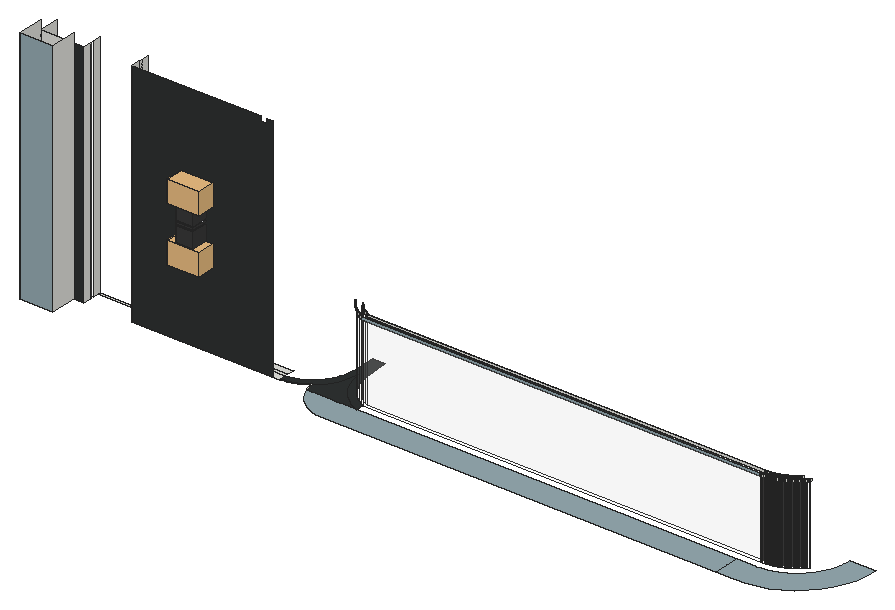
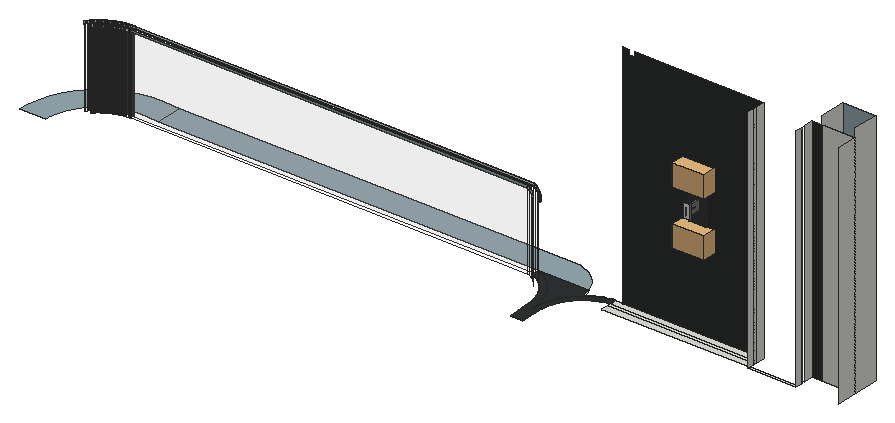
# SketchUp Ruby script. Lengths in inches.
U = 1.inch
M = Sketchup.active_model
def pt(a) = Geom::Point3d.new(a.map { |v| v * U })
def face(e, loops, mat)
  f = e.add_face(loops[0].map { |a| pt(a) })
  loops[1..].each { |l| e.add_face(l.map { |a| pt(a) }).erase! }
  f.material = f.back_material = mat if mat
  f
end
# faces: each face lists its corners as indices into pts; further lists are holes
def faces(e, pts, list, mat = nil) = list.each { |f| face(e, (f[0].is_a?(Array) ? f : [f]).map { |l| l.map { |i| pts[i] } }, mat) }
# xy, xz, yz: faces in a plane at the given z, y or x. An outline is a flat list of corners, or four numbers for a rectangle; further outlines are holes
def ring(l) = l.size == 4 ? [[l[0], l[1]], [l[2], l[1]], [l[2], l[3]], [l[0], l[3]]] : l.each_slice(2).to_a
def flat(e, list, mat, &to3) = list.each { |f| face(e, (f[0].is_a?(Array) ? f : [f]).map { |l| ring(l).map { |u, v| to3.(u, v) } }, mat) }
def xy(e, z, list, mat = nil) = flat(e, list, mat) { |x, y| [x, y, z] }
def xz(e, y, list, mat = nil) = flat(e, list, mat) { |x, z| [x, y, z] }
def yz(e, x, list, mat = nil) = flat(e, list, mat) { |y, z| [x, y, z] }
def lines(e, pts, list) = list.each { |a, b| e.add_line(pt(pts[a]), pt(pts[b])) }
# prism: a flat outline (further loops are holes) pulled along v
def prism(e, loops, v, mat = nil)
  f = face(e, loops, mat); d = Geom::Vector3d.new(v.map { |x| x * U })
  f.pushpull(f.normal.samedirection?(d) ? d.length : -d.length)
end
def box(e, o, s, mat = nil) = prism(e, [[o, [o[0] + s[0], o[1], o[2]], [o[0] + s[0], o[1] + s[1], o[2]], [o[0], o[1] + s[1], o[2]]]], [0, 0, s[2]], mat)
def at(x, y, z, deg = 0) = Geom::Transformation.translation(pt([x, y, z])) * Geom::Transformation.rotation(ORIGIN, Z_AXIS, deg.degrees)
def axes(o, x, y, z) = Geom::Transformation.new([*x, 0, *y, 0, *z, 0, *pt(o).to_a, 1])
def part(name) = M.definitions.add(name)
# library, detail: a bought-in or finely detailed component or shape, given as its bounding box
def library(name, o, s) = part(name).tap { |d| box(d.entities, o, s) }
def detail(e, o, s) = box(e.add_group.entities, o, s)
def put(e, d, t, mat = nil) = e.add_instance(d, t).tap { |i| i.material = mat if mat }
def group(e, t, mat = nil) = e.add_group.tap { |g| g.transformation = t; g.material = mat if mat }.entities
root = M.entities
M.materials.add("11.free-metal-textures").color = [58, 58, 58]
M.materials.add("Generic").color = [150, 171, 178]
M.materials.add("Generic\#1").color = [47, 50, 50]
M.materials.add("Glass Thin Clear 001").color = [252, 250, 250]
M.materials["Glass Thin Clear 001"].alpha = 0.1
M.materials.add("[0111_SlateGray]").color = [112, 128, 144]
M.materials.add("[0117_GhostWhite]").color = [248, 248, 255]
M.materials.add("images").color = [124, 124, 124]
c1 = library("Spot Light",[-7.3,-7.3,-9.9375],[14.6,14.6,9.9375])
c2 = part("Group0\#1")
p = [[-17.97,0.98,0],[-6.48,-16.79,0],[0,0,38],[13.97,-11.35,0],[15.11,9.78,0],[-4.625,17.4,0]]
faces(c2.entities,p,[[0,1,2],[1,3,2],[3,4,2],[5,0,2],[4,5,2]])
c3 = part("wall light")
g1 = group(c3.entities,at(188.14,62.59,-1.03))
xy(g1,0.24,[[[0,0,7.875,7.875],[0.49,0.49,7.38,7.38]]],"images")
xy(g1,1.03,[[[0.49,0.49,7.38,7.38],[0.73,0.73,7.14,7.14]]],"[0111_SlateGray]")
xy(g1,2.21,[[0.73,0.73,7.14,7.14]],"[0117_GhostWhite]")
xy(g1,5.75,[[2.36,13.78,5.51,14.17]],"images")
xy(g1,6.74,[[3.35,7.875,4.52,13.78]],"images")
xy(g1,7.72,[[0,0,7.875,0,7.875,7.875,7.38,7.875,7.38,0.49,0.49,0.49,0.49,7.875,0,7.875],[0.49,7.38,7.38,7.875]])
xy(g1,8.5,[[3.35,9.63,4.52,12.02]])
xy(g1,8.51,[[0,0,0,7.875,0.49,7.875,0.49,0.49,7.38,0.49,7.38,7.875,7.875,7.875,7.875,0]])
xy(g1,9.29,[[0,0,7.875,0,7.875,7.875,7.38,7.875,7.38,0.49,0.49,0.49,0.49,7.875,0,7.875]])
xy(g1,9.3,[[3.35,9.63,4.52,12.02]])
xy(g1,10.08,[[0,0,7.875,0,7.875,7.875,7.38,7.875,7.38,0.49,0,0.49],[0,0.49,0.49,7.875],[0.49,7.38,7.38,7.875]])
xy(g1,11.06,[[3.35,7.875,4.52,13.78]],"images")
xy(g1,12.05,[[2.36,13.78,5.51,14.17]],"images")
xy(g1,15.59,[[0.73,0.73,7.14,7.14]],"[0117_GhostWhite]")
xy(g1,16.77,[[[0.49,0.49,7.38,7.38],[0.73,0.73,7.14,7.14]]],"[0111_SlateGray]")
xy(g1,17.5625,[[[0,0,7.875,7.875],[0.49,0.49,7.38,7.38]]],"images")
xz(g1,0,[[0,0.24,7.875,7.72],[0,8.51,7.875,9.29],[0,10.08,7.875,17.5625]],"11.free-metal-textures")
xz(g1,0.49,[[0.49,8.51,7.38,8.9],[0.49,8.9,7.38,9.29]])
xz(g1,0.49,[[0.49,0.24,7.38,1.03],[0.49,16.77,7.38,17.5625]],"[0111_SlateGray]")
xz(g1,0.49,[[0.49,7.72,7.38,8.51],[0.49,9.29,7.38,10.08]],"[0117_GhostWhite]")
xz(g1,0.73,[[0.73,1.03,7.14,2.21],[0.73,2.21,7.14,15.59],[0.73,15.59,7.14,16.77]],"[0111_SlateGray]")
xz(g1,7.14,[[0.73,1.03,7.14,2.21],[0.73,2.21,7.14,15.59],[0.73,15.59,7.14,16.77]],"[0111_SlateGray]")
xz(g1,7.38,[[0.49,0.24,7.38,1.03],[0.49,16.77,7.38,17.5625]],"[0111_SlateGray]")
xz(g1,7.875,[[3.35,6.74,4.52,7.72],[3.35,7.72,3.9375,10.08],[3.9375,7.72,4.52,10.08],[3.35,10.08,4.52,11.06]])
xz(g1,7.875,[[0,0.24,0,7.72,3.35,7.72,3.35,6.74,4.52,6.74,4.52,7.72,7.875,7.72,7.875,0.24],[0.49,7.72,0.49,8.51,0,8.51,0,9.29,0.49,9.29,0.49,10.08,3.35,10.08,3.35,7.72],[4.52,7.72,4.52,10.08,7.38,10.08,7.38,9.29,7.875,9.29,7.875,8.51,7.38,8.51,7.38,7.72],[0,10.08,0,17.5625,7.875,17.5625,7.875,10.08,4.52,10.08,4.52,11.06,3.35,11.06,3.35,10.08]],"11.free-metal-textures")
xz(g1,9.63,[[3.35,8.5,4.52,9.3]])
xz(g1,12.02,[[3.35,8.5,4.52,9.3]])
xz(g1,13.78,[[2.36,5.75,4.52,5.75,4.52,6.74,3.35,6.74,3.35,11.06,4.52,11.06,4.52,5.75,5.51,5.75,5.51,12.05,2.36,12.05]],"images")
xz(g1,14.17,[[2.36,5.75,5.51,12.05]])
yz(g1,0,[[0,0.24,7.875,7.72],[0,8.51,7.875,9.29],[0,10.08,7.875,17.5625]],"11.free-metal-textures")
yz(g1,0.49,[[0.49,8.51,7.38,8.9]])
yz(g1,0.49,[[0.49,0.24,7.38,1.03],[0.49,16.77,7.38,17.5625]],"[0111_SlateGray]")
yz(g1,0.49,[[0.49,7.72,7.875,8.51],[0.49,9.29,7.875,10.08]],"[0117_GhostWhite]")
yz(g1,0.73,[[0.73,1.03,7.14,2.21],[0.73,2.21,7.14,15.59],[0.73,15.59,7.14,16.77]],"[0111_SlateGray]")
yz(g1,2.36,[[13.78,5.75,14.17,12.05]],"images")
yz(g1,3.35,[[[7.875,6.74,13.78,11.06],[9.63,8.5,12.02,9.3]]],"images")
yz(g1,4.52,[[[7.875,6.74,13.78,11.06],[9.63,8.5,12.02,9.3]]],"images")
yz(g1,5.51,[[13.78,5.75,14.17,12.05]],"images")
yz(g1,7.14,[[0.73,1.03,7.14,2.21],[0.73,2.21,7.14,15.59],[0.73,15.59,7.14,16.77]],"[0111_SlateGray]")
yz(g1,7.38,[[0.49,8.51,7.38,8.9]])
yz(g1,7.38,[[0.49,0.24,7.38,1.03],[0.49,16.77,7.38,17.5625]],"[0111_SlateGray]")
yz(g1,7.38,[[0.49,7.72,7.875,8.51],[0.49,9.29,7.875,10.08]],"[0117_GhostWhite]")
yz(g1,7.875,[[0,0.24,7.875,7.72],[0,8.51,7.875,9.29],[0,10.08,7.875,17.5625]],"11.free-metal-textures")
p = [[7.38,7.38,8.9],[0.49,7.38,8.9],[4.52,7.875,6.54],[4.52,7.875,6.74],[4.52,13.78,5.5625],[4.52,13.78,5.75]]
lines(g1,p,[[0,1],[2,3],[4,5]])
put(g1,c2,axes([3.74,4.28,0],[0.1617,0,0],[0,0.1617,0],[0,0,0.1617]))
put(g1,c2,axes([4.15,3.625,18],[-0.1617,0,0],[0,0.1617,0],[0,0,-0.1617]))
xy(root,257,[[10.218,29.933,25.218,42.0625],[51.935,42.0625,119.415,42.0625,119.415,45.199,119.209,45.171,51.935,45.171],[119.415,42.0625,120.438,42.148,121.455,42.289,122.463,42.485,123.459,42.737,124.439,43.042,125.401,43.4,126.342,43.81,127.26,44.271,128.151,44.781,129.013,45.339,129.843,45.943,130.639,46.592,129.741,45.931,128.812,45.317,127.853,44.749,126.867,44.231,125.856,43.763,124.822,43.346,123.769,42.981,122.699,42.67,121.615,42.412,120.52,42.21],[131.803,42.0625,131.538,42.727,130.991,44.637,130.639,46.592,130.68,46.202,130.731,45.814,130.793,45.428,130.865,45.043,130.947,44.661,131.039,44.28,131.142,43.903,131.254,43.528,131.377,43.156,131.509,42.788,131.651,42.423],[51.935,45.171,119.209,45.171,119.415,45.199,119.415,46.971,119.092,46.928,51.935,46.928],
  [51.935,46.928,119.092,46.928,119.415,46.971,119.415,50.209,119.252,50.179,118.879,50.129,51.935,50.129],[29.81,50.129,51.935,51.0625]])
xy(root,257,[[145.638,29.933,328.648,29.933,328.648,42.0625,131.803,42.0625,132.274,40.883,133.193,39.122,134.284,37.462,135.537,35.921,136.939,34.513,138.476,33.255,140.131,32.157,141.889,31.231,143.73,30.488],[328.648,29.933,337.218,29.933,341.984,30.085,346.685,30.887,351.231,32.326,355.538,34.373,359.524,36.991,363.114,40.13,366.24,43.731,368.843,47.726,370.876,52.04,372.298,56.592,373.083,61.296,373.218,66.0625,361.218,66.0625,361.532,66.058,361.523,65.426,361.498,64.79,361.457,64.155,361.399,63.521,361.324,62.889,361.232,62.259,361.125,61.632,361,61.007,360.86,60.386,360.703,59.77,360.531,59.157,360.342,58.549,360.137,57.946,359.917,57.349,359.681,56.758,359.43,56.173,359.163,55.595,358.882,55.024,358.585,54.461,358.274,53.905,357.949,53.358,357.609,52.82,357.256,52.291,356.888,51.771,356.507,51.261,356.113,50.761,355.706,50.272,355.287,49.793,354.854,49.326,354.41,48.87,353.954,48.426,353.487,47.994,353.008,47.574,352.519,47.167,352.019,46.773,351.509,46.392,350.989,46.025,350.46,45.671,349.922,45.331,349.375,45.006,348.819,44.695,348.256,44.398,347.685,44.117,347.107,43.85,346.522,43.599,345.931,43.363,345.334,43.143,344.731,42.938,344.123,42.75,343.511,42.577,342.894,42.42,342.273,42.28,341.648,42.155,341.021,42.048,340.391,41.956,339.759,41.882,339.125,41.823,338.49,41.782,337.854,41.757,337.222,41.748,337.222,42.0625,328.648,42.0625]],"Generic")
xy(root,257,[[119.415,42.0625,120.52,42.21,121.615,42.412,122.699,42.67,123.769,42.981,124.822,43.346,125.856,43.763,126.867,44.231,127.853,44.749,128.812,45.317,129.741,45.931,130.639,46.592,131.502,47.296,132.329,48.043,133.117,48.831,133.865,49.657,134.57,50.52,135.231,51.417,135.846,52.346,136.414,53.304,136.933,54.29,137.402,55.301,137.82,56.334,138.186,57.387,138.498,58.456,138.756,59.54,138.959,60.636,139.107,61.74,139.2,62.851,139.218,63.384,139.218,65.078,139.349,62.635,139.718,60.216,140.322,57.844,141.154,55.543,142.207,53.333,143.47,51.238,144.932,49.275,146.578,47.464,148.394,45.823,150.36,44.367,152.46,43.109,154.672,42.0625,154.672,45.502,153.927,45.854,152.088,46.955,150.366,48.231,148.776,49.668,147.334,51.254,146.054,52.973,144.948,54.808,144.026,56.743,143.297,58.758,142.769,60.835,142.445,62.954,141.834,74.3125,136.109,74.3125,136.109,63.436,136.096,63.031,136.016,62.076,135.889,61.127,135.714,60.184,135.492,59.252,135.223,58.332,134.909,57.427,134.55,56.539,134.146,55.67,133.7,54.822,133.212,53.997,132.682,53.198,132.114,52.427,131.507,51.685,130.864,50.975,130.187,50.298,129.476,49.655,128.733,49.049,127.962,48.481,127.162,47.953,126.338,47.465,125.489,47.019,124.62,46.616,123.731,46.258,122.826,45.944,121.906,45.676,120.973,45.455,120.031,45.281,119.415,45.199],[131.803,42.0625,154.672,42.0625,152.46,43.109,150.36,44.367,148.394,45.823,146.578,47.464,144.932,49.275,143.47,51.238,142.207,53.333,141.154,55.543,140.322,57.844,139.718,60.216,139.349,62.635,139.218,65.078,139.237,63.964,139.218,63.384,139.2,62.851,139.107,61.74,138.959,60.636,138.756,59.54,138.498,58.456,138.186,57.387,137.82,56.334,137.402,55.301,136.933,54.29,136.414,53.304,135.846,52.346,135.231,51.417,134.57,50.52,133.865,49.657,133.117,48.831,132.329,48.043,131.502,47.296,130.639,46.592,130.991,44.637,131.538,42.727]],"Generic\#1")
xz(root,29.933,[[10.218,257,25.218,366]],"Generic")
xz(root,42.0625,[[10.218,257,25.218,362]])
xz(root,42.0625,[[25.218,257,29.81,362],[51.935,257,116.202,257,116.202,362,113.607,362,113.607,360,111.013,360,111.013,362,51.935,362]],"Generic\#1")
xz(root,44.615,[[155.245,293,337.201,294]],"Generic")
xz(root,44.796,[[155.286,293,337.2,294]])
xz(root,45.171,[[155.37,257,337.197,293]],"Glass Thin Clear 001")
xz(root,46.928,[[155.765,257,337.186,293]],"Glass Thin Clear 001")
xz(root,47.303,[[155.849,293,337.183,294]])
xz(root,47.484,[[155.889,293,337.182,294]],"Generic")
yz(root,10.218,[[29.933,257,42.0625,366],[42.0625,257,51.0625,362]])
yz(root,25.218,[[29.933,257,42.0625,366]])
yz(root,29.81,[[42.0625,257,46.096,362],[47.721,257,51.0625,362]])
yz(root,29.81,[[46.096,257,47.721,362]],"Glass Thin Clear 001")
yz(root,51.935,[[42.0625,257,46.096,362],[46.096,257,47.721,362],[47.721,257,51.0625,362]])
p = [[153.927,45.854,257],[154.672,45.502,257],[155.37,45.171,257],[155.37,45.171,293],[153.927,45.854,293],[337.197,45.171,257],
  [337.764,45.179,257],[337.764,45.179,293],[337.197,45.171,293],[338.311,45.2,257],[338.311,45.2,293],[338.857,45.236,257],
  [338.857,45.236,293],[339.468,45.292,257],[339.468,45.292,293],[339.902,45.3,257],[339.902,45.3,293],[340.186,45.333,257],
  [340.186,45.333,293],[340.592,45.389,257],[340.592,45.389,293],[340.996,45.453,257],[340.996,45.453,293],[341.399,45.525,257],
  [341.399,45.525,293],[341.801,45.605,257],[341.801,45.605,293],[342.201,45.693,257],[342.201,45.693,293],[342.599,45.789,257],
  [342.599,45.789,293],[342.995,45.893,257],[342.995,45.893,293],[152.088,46.955,257],[152.088,46.955,293],[343.389,46.004,257],
  [343.389,46.004,293],[343.781,46.124,257],[343.781,46.124,293],[344.17,46.251,257],[344.17,46.251,293],[344.557,46.387,257],
  [344.557,46.387,293],[344.941,46.529,257],[344.941,46.529,293],[345.322,46.68,257],[345.322,46.68,293],[345.699,46.838,257],
  [345.699,46.838,293],[346.074,47.003,257],[346.074,47.003,293],[155.765,46.928,257],[154.755,47.405,257],[154.755,47.405,293],
  [155.765,46.928,293],[337.718,46.935,257],[337.186,46.928,257],[337.186,46.928,293],[337.718,46.935,293],[338.219,46.954,257],
  [338.219,46.954,293],[150.366,48.231,257],[150.366,48.231,293],[338.719,46.987,257],[338.719,46.987,293],[339.372,47.047,257],
  [339.372,47.047,293],[339.784,47.054,257],[339.784,47.054,293],[346.445,47.176,257],[346.445,47.176,293],[339.964,47.075,257],
  [339.964,47.075,293],[340.335,47.127,257],[340.335,47.127,293],[340.705,47.185,257],[340.705,47.185,293],[341.073,47.251,257],
  [341.073,47.251,293],[346.813,47.357,257],[346.813,47.357,293],[341.441,47.324,257],[341.441,47.324,293],[341.806,47.404,257],
  [341.806,47.404,293],[154.672,47.455,257],[153.064,48.418,257],[153.064,48.418,293],[342.171,47.492,257],[342.171,47.492,293],
  [347.177,47.545,257],[347.177,47.545,293],[342.533,47.587,257],[342.533,47.587,293],[347.537,47.739,257],[347.537,47.739,293],
  [342.893,47.689,257],[342.893,47.689,293],[343.251,47.799,257],[343.251,47.799,293],[347.893,47.941,257],[347.893,47.941,293],
  [343.607,47.915,257],[343.607,47.915,293],[343.961,48.039,257],[343.961,48.039,293],[348.245,48.151,257],[348.245,48.151,293],
  [344.312,48.169,257],[344.312,48.169,293],[148.776,49.668,257],[148.776,49.668,293],[344.66,48.307,257],[344.66,48.307,293],
  [348.593,48.367,257],[348.593,48.367,293],[345.005,48.452,257],[345.005,48.452,293],[151.48,49.591,257],[151.48,49.591,293],
  [348.937,48.59,257],[348.937,48.59,293],[345.348,48.603,257],[345.348,48.603,293],[345.6875,48.761,257],[345.6875,48.761,293],
  [349.276,48.82,257],[349.276,48.82,293],[346.024,48.926,257],[346.024,48.926,293],[349.61,49.056,257],[349.61,49.056,293],
  [346.356,49.098,257],[346.356,49.098,293],[346.686,49.276,257],[346.686,49.276,293],[349.94,49.299,257],[349.94,49.299,293],
  [347.011,49.461,257],[347.011,49.461,293],[350.264,49.549,257],[350.264,49.549,293],[347.333,49.652,257],[347.333,49.652,293],
  [350.584,49.805,257],[350.584,49.805,293],[150.018,50.913,257],[150.018,50.913,293],[147.334,51.254,257],[147.334,51.254,293],
  [347.652,49.849,257],[347.652,49.849,293],[347.966,50.053,257],[347.966,50.053,293],[350.898,50.068,257],[350.898,50.068,293],
  [348.276,50.264,257],[348.276,50.264,293],[351.207,50.336,257],[351.207,50.336,293],[348.581,50.48,257],[348.581,50.48,293],
  [351.511,50.611,257],[351.511,50.611,293],[348.883,50.702,257],[348.883,50.702,293],[351.809,50.892,257],[351.809,50.892,293],
  [349.179,50.931,257],[349.179,50.931,293],[148.692,52.372,257],[148.692,52.372,293],[349.472,51.165,257],[349.472,51.165,293],
  [352.102,51.178,257],[352.102,51.178,293],[349.759,51.405,257],[349.759,51.405,293],[352.388,51.471,257],[352.388,51.471,293],
  [146.054,52.973,257],[146.054,52.973,293],[350.042,51.65,257],[350.042,51.65,293],[352.669,51.769,257],[352.669,51.769,293],
  [350.32,51.902,257],[350.32,51.902,293],[352.944,52.073,257],[352.944,52.073,293],[350.592,52.158,257],[350.592,52.158,293],
  [353.213,52.382,257],[353.213,52.382,293],[350.86,52.421,257],[350.86,52.421,293],[351.122,52.688,257],[351.122,52.688,293],
  [353.475,52.696,257],[353.475,52.696,293],[351.378,52.961,257],[351.378,52.961,293],[353.731,53.016,257],[353.731,53.016,293],
  [153.664,45.363,294],[153.664,45.363,293],[155.245,44.615,293],[155.245,44.615,294],[337.201,44.615,294],[337.201,44.615,293],
  [337.779,44.623,293],[337.779,44.623,294],[338.34,44.645,293],[338.34,44.645,294],[338.9,44.681,293],[338.9,44.681,294],
  [339.499,44.736,293],[339.499,44.736,294],[339.939,44.744,293],[339.939,44.744,294],[340.256,44.781,293],[340.256,44.781,294],
  [155.286,44.796,293],[155.286,44.796,294],[153.75,45.523,294],[153.75,45.523,293],[337.774,44.804,293],[337.774,44.804,294],
  [337.2,44.796,294],[337.2,44.796,293],[338.331,44.826,293],[338.331,44.826,294],[338.886,44.862,293],[338.886,44.862,294],
  [340.673,44.839,293],[340.673,44.839,294],[341.088,44.904,293],[341.088,44.904,294],[339.489,44.917,293],[339.489,44.917,294],
  [339.927,44.925,293],[339.927,44.925,294],[340.233,44.961,293],[340.233,44.961,294],[341.503,44.978,293],[341.503,44.978,294],
  [340.647,45.018,293],[340.647,45.018,294],[341.058,45.083,293],[341.058,45.083,294],[341.915,45.06,293],[341.915,45.06,294],
  [341.469,45.156,293],[341.469,45.156,294],[342.326,45.151,293],[342.326,45.151,294],[341.878,45.238,293],[341.878,45.238,294],
  [342.285,45.327,293],[342.285,45.327,294],[342.735,45.249,293],[342.735,45.249,294],[343.142,45.356,293],[343.142,45.356,294],
  [342.691,45.425,293],[342.691,45.425,294],[151.779,46.492,294],[151.779,46.492,293],[343.094,45.531,293],[343.094,45.531,294],
  [343.546,45.471,293],[343.546,45.471,294],[151.88,46.643,294],[151.88,46.643,293],[343.495,45.645,293],[343.495,45.645,294],
  [343.949,45.594,293],[343.949,45.594,294],[343.894,45.766,293],[343.894,45.766,294],[344.348,45.725,293],[344.348,45.725,294],
  [344.746,45.863,293],[344.746,45.863,294],[344.29,45.896,293],[344.29,45.896,294],[344.684,46.034,293],[344.684,46.034,294],
  [345.14,46.01,293],[345.14,46.01,294],[345.075,46.179,293],[345.075,46.179,294],[345.531,46.165,293],[345.531,46.165,294],
  [345.463,46.332,293],[345.463,46.332,294],[345.919,46.327,293],[345.919,46.327,294],[345.848,46.493,293],[345.848,46.493,294],
  [346.304,46.497,293],[346.304,46.497,294],[150.013,47.8,294],[150.013,47.8,293],[346.229,46.662,293],[346.229,46.662,294],
  [346.685,46.675,293],[346.685,46.675,294],[150.128,47.94,294],[150.128,47.94,293],[346.607,46.838,293],[346.607,46.838,294],
  [347.063,46.86,293],[347.063,46.86,294],[346.981,47.022,293],[346.981,47.022,294],[347.437,47.053,293],[347.437,47.053,294],
  [347.352,47.213,293],[347.352,47.213,294],[347.807,47.253,293],[347.807,47.253,294],[347.719,47.411,293],[347.719,47.411,294],
  [154.932,47.736,293],[154.932,47.736,294],[155.849,47.303,294],[155.849,47.303,293],[337.183,47.303,293],[337.183,47.303,294],
  [337.709,47.31,294],[337.709,47.31,293],[338.199,47.329,294],[338.199,47.329,293],[338.689,47.361,294],[338.689,47.361,293],
  [348.172,47.461,293],[348.172,47.461,294],[339.352,47.422,294],[339.352,47.422,293],[339.759,47.429,294],[339.759,47.429,293],
  [339.917,47.447,294],[339.917,47.447,293],[340.28,47.497,294],[340.28,47.497,293],[348.082,47.617,293],[348.082,47.617,294],
  [155.889,47.484,294],[155.889,47.484,293],[155.018,47.896,293],[155.018,47.896,294],[337.704,47.491,294],[337.704,47.491,293],
  [337.182,47.484,293],[337.182,47.484,294],[338.19,47.51,294],[338.19,47.51,293],[338.675,47.541,294],[338.675,47.541,293],
  [339.342,47.603,294],[339.342,47.603,293],[340.643,47.555,294],[340.643,47.555,293],[348.534,47.675,293],[348.534,47.675,294],
  [339.746,47.61,294],[339.746,47.61,293],[339.894,47.627,294],[339.894,47.627,293],[340.254,47.677,294],[340.254,47.677,293],
  [341.004,47.619,294],[341.004,47.619,293],[341.364,47.691,294],[341.364,47.691,293],[348.44,47.83,293],[348.44,47.83,294],
  [153.273,48.73,293],[153.273,48.73,294],[340.613,47.733,294],[340.613,47.733,293],[340.97,47.797,294],[340.97,47.797,293],
  [341.722,47.77,294],[341.722,47.77,293],[348.891,47.897,293],[348.891,47.897,294],[148.383,49.274,294],[148.383,49.274,293],
  [341.327,47.868,294],[341.327,47.868,293],[342.079,47.856,294],[342.079,47.856,293],[348.794,48.05,293],[348.794,48.05,294],
  [148.511,49.402,294],[148.511,49.402,293],[153.373,48.881,293],[153.373,48.881,294],[341.682,47.946,294],[341.682,47.946,293],
  [342.035,48.031,294],[342.035,48.031,293],[342.434,47.949,294],[342.434,47.949,293],[342.787,48.049,294],[342.787,48.049,293],
  [349.244,48.126,293],[349.244,48.126,294],[342.386,48.124,294],[342.386,48.124,293],[343.138,48.156,294],[343.138,48.156,293],
  [342.736,48.223,294],[342.736,48.223,293],[349.144,48.277,293],[349.144,48.277,294],[349.592,48.362,293],[349.592,48.362,294],
  [343.083,48.329,294],[343.083,48.329,293],[343.487,48.27,294],[343.487,48.27,293],[343.429,48.442,294],[343.429,48.442,293],
  [343.833,48.392,294],[343.833,48.392,293],[349.489,48.511,293],[349.489,48.511,294],[343.772,48.562,294],[343.772,48.562,293],
  [344.177,48.52,294],[344.177,48.52,293],[349.936,48.605,293],[349.936,48.605,294],[344.519,48.654,294],[344.519,48.654,293],
  [349.83,48.752,293],[349.83,48.752,294],[344.112,48.689,294],[344.112,48.689,293],[350.274,48.855,293],[350.274,48.855,294],
  [151.718,49.882,293],[151.718,49.882,294],[344.45,48.822,294],[344.45,48.822,293],[344.857,48.796,294],[344.857,48.796,293],
  [344.786,48.962,294],[344.786,48.962,293],[345.193,48.944,294],[345.193,48.944,293],[350.165,49,293],[350.165,49,294],
  [151.833,50.022,293],[151.833,50.022,294],[345.526,49.099,294],[345.526,49.099,293],[350.608,49.112,293],[350.608,49.112,294],
  [345.118,49.109,294],[345.118,49.109,293],[350.496,49.254,293],[350.496,49.254,294],[345.447,49.263,294],[345.447,49.263,293],
  [345.855,49.261,294],[345.855,49.261,293],[350.936,49.375,293],[350.936,49.375,294],[146.905,50.9,294],[146.905,50.9,293],
  [345.774,49.423,294],[345.774,49.423,293],[346.181,49.429,294],[346.181,49.429,293],[350.821,49.515,293],[350.821,49.515,294],
  [147.045,51.015,294],[147.045,51.015,293],[346.097,49.589,294],[346.097,49.589,293],[346.504,49.604,294],[346.504,49.604,293],
  [351.259,49.644,293],[351.259,49.644,294],[351.141,49.782,293],[351.141,49.782,294],[346.416,49.762,294],[346.416,49.762,293],
  [346.823,49.785,294],[346.823,49.785,293],[351.576,49.92,293],[351.576,49.92,294],[346.732,49.942,294],[346.732,49.942,293],
  [347.139,49.972,294],[347.139,49.972,293],[351.456,50.056,293],[351.456,50.056,294],[150.283,51.179,293],[150.283,51.179,294],
  [347.045,50.127,294],[347.045,50.127,293],[351.888,50.202,293],[351.888,50.202,294],[150.411,51.308,293],[150.411,51.308,294],
  [347.45,50.166,294],[347.45,50.166,293],[347.353,50.319,294],[347.353,50.319,293],[351.765,50.335,293],[351.765,50.335,294],
  [347.758,50.366,294],[347.758,50.366,293],[352.194,50.491,293],[352.194,50.491,294],[347.658,50.517,294],[347.658,50.517,293],
  [352.069,50.621,293],[352.069,50.621,294],[348.062,50.572,294],[348.062,50.572,293],[347.959,50.721,294],[347.959,50.721,293],
  [352.495,50.785,293],[352.495,50.785,294],[348.362,50.784,294],[348.362,50.784,293],[352.367,50.913,293],[352.367,50.913,294],
  [348.256,50.931,294],[348.256,50.931,293],[348.657,51.002,294],[348.657,51.002,293],[352.789,51.086,293],[352.789,51.086,294],
  [145.592,52.662,294],[145.592,52.662,293],[348.548,51.146,294],[348.548,51.146,293],[352.659,51.211,293],[352.659,51.211,294],
  [145.742,52.763,294],[145.742,52.763,293],[348.948,51.225,294],[348.948,51.225,293],[348.836,51.368,294],[348.836,51.368,293],
  [353.078,51.392,293],[353.078,51.392,294],[148.982,52.611,293],[148.982,52.611,294],[349.234,51.455,294],[349.234,51.455,293],
  [352.945,51.515,293],[352.945,51.515,294],[149.121,52.726,293],[149.121,52.726,294],[349.12,51.595,294],[349.12,51.595,293],
  [353.36,51.704,293],[353.36,51.704,294],[349.516,51.69,294],[349.516,51.69,293],[353.224,51.824,293],[353.224,51.824,294],
  [349.399,51.828,294],[349.399,51.828,293],[349.793,51.931,294],[349.793,51.931,293],[353.636,52.021,293],[353.636,52.021,294],
  [349.673,52.066,294],[349.673,52.066,293],[353.498,52.139,293],[353.498,52.139,294],[350.065,52.177,294],[350.065,52.177,293],
  [353.905,52.344,293],[353.905,52.344,294],[349.942,52.31,294],[349.942,52.31,293],[353.765,52.459,293],[353.765,52.459,294],
  [350.332,52.429,294],[350.332,52.429,293],[350.207,52.559,294],[350.207,52.559,293],[354.169,52.672,293],[354.169,52.672,294],
  [350.594,52.686,294],[350.594,52.686,293],[354.026,52.784,293],[354.026,52.784,294],[350.466,52.814,294],[350.466,52.814,293],
  [350.851,52.948,294],[350.851,52.948,293],[354.425,53.006,293],[354.425,53.006,294],[350.721,53.073,294],[350.721,53.073,293],
  [354.28,53.115,293],[354.28,53.115,294]]
faces(root,p,[[0,1,2,3,4],[5,6,7,8],[6,9,10,7],[9,11,12,10],[11,13,14,12],[13,15,16,14],[15,17,18,16],[17,19,20,18],
  [19,21,22,20],[21,23,24,22],[23,25,26,24],[25,27,28,26],[27,29,30,28],[29,31,32,30],[33,0,4,34],[31,35,36,32],
  [35,37,38,36],[37,39,40,38],[39,41,42,40],[41,43,44,42],[43,45,46,44],[45,47,48,46],[47,49,50,48],[51,52,53,54],
  [55,56,57,58],[59,55,58,60],[61,33,34,62],[63,59,60,64],[65,63,64,66],[67,65,66,68],[49,69,70,50],[71,67,68,72],
  [73,71,72,74],[75,73,74,76],[77,75,76,78],[69,79,80,70],[81,77,78,82],[83,81,82,84],[85,86,87,53,52],[88,83,84,89],
  [79,90,91,80],[92,88,89,93],[90,94,95,91],[96,92,93,97],[98,96,97,99],[94,100,101,95],[102,98,99,103],[104,102,103,105],
  [100,106,107,101],[108,104,105,109],[110,61,62,111],[112,108,109,113],[106,114,115,107],[116,112,113,117],[86,118,119,87],[114,120,121,115],
  [122,116,117,123],[124,122,123,125],[120,126,127,121],[128,124,125,129],[126,130,131,127],[132,128,129,133],[134,132,133,135],[130,136,137,131],
  [138,134,135,139],[136,140,141,137],[142,138,139,143],[140,144,145,141],[118,146,147,119],[148,110,111,149],[150,142,143,151],[152,150,151,153],
  [144,154,155,145],[156,152,153,157],[154,158,159,155],[160,156,157,161],[158,162,163,159],[164,160,161,165],[162,166,167,163],[168,164,165,169],
  [146,170,171,147],[172,168,169,173],[166,174,175,167],[176,172,173,177],[174,178,179,175],[180,148,149,181],[182,176,177,183],[178,184,185,179],
  [186,182,183,187],[184,188,189,185],[190,186,187,191],[188,192,193,189],[194,190,191,195],[196,194,195,197],[192,198,199,193],[200,196,197,201],
  [198,202,203,199]],"Glass Thin Clear 001")
faces(root,p,[[204,205,206,207],[208,209,210,211],[211,210,212,213],[213,212,214,215],[215,214,216,217],[217,216,218,219],[219,218,220,221],[222,223,224,225],
  [226,227,228,229],[230,231,227,226],[232,233,231,230],[221,220,234,235],[235,234,236,237],[238,239,233,232],[240,241,239,238],[242,243,241,240],
  [237,236,244,245],[246,247,243,242],[248,249,247,246],[245,244,250,251],[252,253,249,248],[251,250,254,255],[256,257,253,252],[258,259,257,256],
  [255,254,260,261],[261,260,262,263],[264,265,259,258],[266,267,205,204],[268,269,265,264],[263,262,270,271],[225,224,272,273],[274,275,269,268],
  [271,270,276,277],[278,279,275,274],[277,276,280,281],[281,280,282,283],[284,285,279,278],[286,287,285,284],[283,282,288,289],[290,291,287,286],
  [289,288,292,293],[294,295,291,290],[293,292,296,297],[298,299,295,294],[297,296,300,301],[302,303,267,266],[304,305,299,298],[301,300,306,307],
  [273,272,308,309],[310,311,305,304],[307,306,312,313],[314,315,311,310],[313,312,316,317],[318,319,315,314],[317,316,320,321],[322,323,319,318],
  [324,325,326,327],[328,329,330,331],[331,330,332,333],[333,332,334,335],[321,320,336,337],[335,334,338,339],[339,338,340,341],[341,340,342,343],
  [343,342,344,345],[346,347,323,322],[348,349,350,351],[352,353,354,355],[356,357,353,352],[358,359,357,356],[360,361,359,358],[345,344,362,363],
  [337,336,364,365],[366,367,361,360],[368,369,367,366],[370,371,369,368],[363,362,372,373],[373,372,374,375],[376,377,347,346],[378,379,325,324],
  [380,381,371,370],[382,383,381,380],[375,374,384,385],[365,364,386,387],[388,389,303,302],[390,391,383,382],[385,384,392,393],[394,395,377,376],
  [309,308,396,397],[351,350,398,399],[400,401,391,390],[402,403,401,400],[393,392,404,405],[405,404,406,407],[387,386,408,409],[410,411,403,402],
  [407,406,412,413],[414,415,411,410],[416,417,395,394],[409,408,418,419],[420,421,415,414],[413,412,422,423],[424,425,421,420],[423,422,426,427],
  [428,429,417,416],[430,431,425,424],[427,426,432,433],[419,418,434,435],[433,432,436,437],[438,439,429,428],[440,441,431,430],[435,434,442,443],
  [444,445,379,378],[446,447,441,440],[437,436,448,449],[450,451,447,446],[449,448,452,453],[454,455,439,438],[399,398,456,457],[453,452,458,459],
  [443,442,460,461],[462,463,451,450],[464,465,455,454],[466,467,463,462],[459,458,468,469],[461,460,470,471],[472,473,389,388],[474,475,467,466],
  [469,468,476,477],[478,479,465,464],[397,396,480,481],[482,483,475,474],[477,476,484,485],[471,470,486,487],[488,489,479,478],[490,491,483,482],
  [485,484,492,493],[487,486,494,495],[496,497,491,490],[493,492,498,499],[500,501,489,488],[502,503,445,444],[504,505,497,496],[495,494,506,507],
  [457,456,508,509],[499,498,510,511],[512,513,505,504],[514,515,501,500],[511,510,516,517],[507,506,518,519],[520,521,513,512],[522,523,515,514],
  [517,516,524,525],[526,527,521,520],[519,518,528,529],[525,524,530,531],[532,533,523,522],[534,535,527,526],[531,530,536,537],[529,528,538,539],
  [540,541,473,472],[542,543,535,534],[544,545,533,532],[481,480,546,547],[537,536,548,549],[550,551,543,542],[539,538,552,553],[554,555,503,502],
  [549,548,556,557],[558,559,545,544],[509,508,560,561],[562,563,551,550],[553,552,564,565],[557,556,566,567],[568,569,559,558],[570,571,563,562],
  [567,566,572,573],[565,564,574,575],[576,577,571,570],[578,579,569,568],[573,572,580,581],[575,574,582,583],[584,585,577,576],[586,587,579,578],
  [581,580,588,589],[590,591,585,584],[583,582,592,593],[589,588,594,595],[596,597,587,586],[598,599,591,590],[595,594,600,601],[593,592,602,603],
  [604,605,599,598],[606,607,597,596]])
put(root,c1,at(81.74,41,301.99))
put(root,c1,axes([81.74,41,317.16],[1,0,0],[0,1,0],[0,0,-1]))
put(root,c3,at(-110.42,-27.91,302.09))
